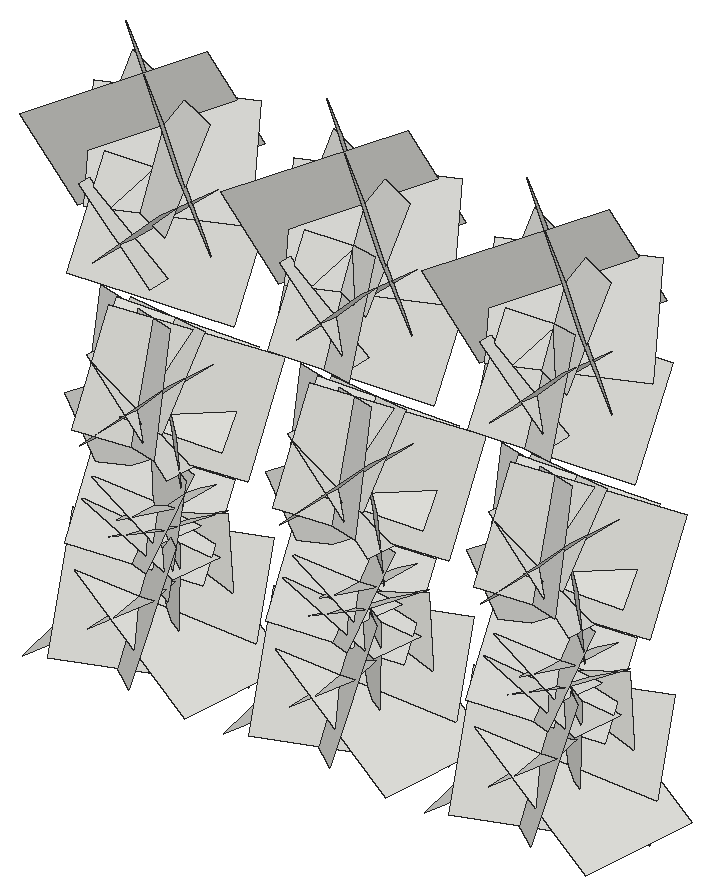
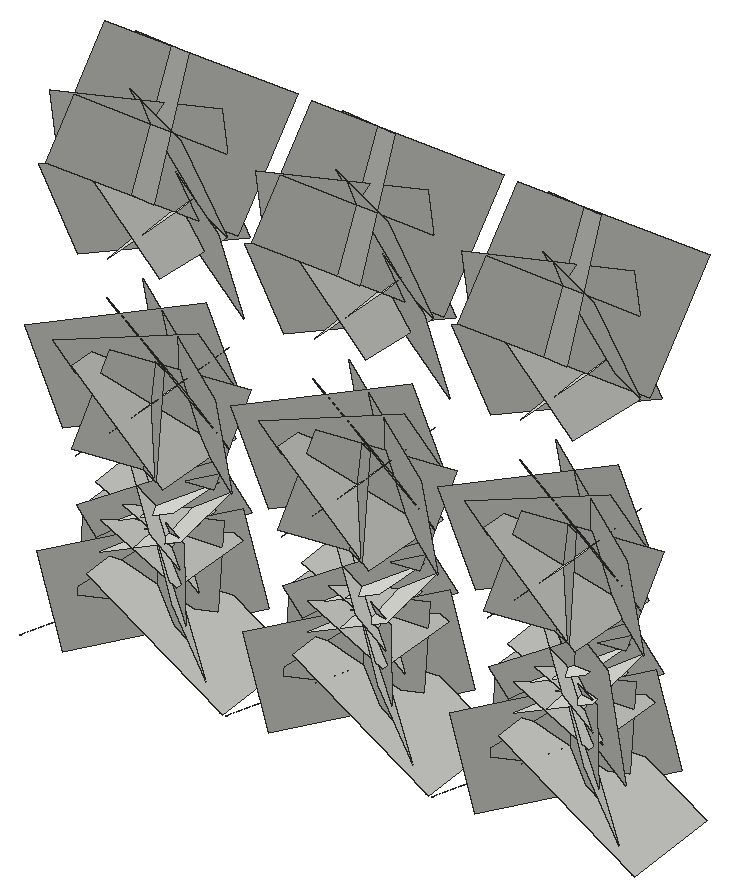
# SketchUp Ruby script. Lengths in inches.
U = 1.inch
M = Sketchup.active_model
def pt(a) = Geom::Point3d.new(a.map { |v| v * U })
def face(e, loops, mat)
  f = e.add_face(loops[0].map { |a| pt(a) })
  loops[1..].each { |l| e.add_face(l.map { |a| pt(a) }).erase! }
  f.material = f.back_material = mat if mat
  f
end
# faces: each face lists its corners as indices into pts; further lists are holes
def faces(e, pts, list, mat = nil) = list.each { |f| face(e, (f[0].is_a?(Array) ? f : [f]).map { |l| l.map { |i| pts[i] } }, mat) }
# xy, xz, yz: faces in a plane at the given z, y or x. An outline is a flat list of corners, or four numbers for a rectangle; further outlines are holes
def ring(l) = l.size == 4 ? [[l[0], l[1]], [l[2], l[1]], [l[2], l[3]], [l[0], l[3]]] : l.each_slice(2).to_a
def flat(e, list, mat, &to3) = list.each { |f| face(e, (f[0].is_a?(Array) ? f : [f]).map { |l| ring(l).map { |u, v| to3.(u, v) } }, mat) }
def xy(e, z, list, mat = nil) = flat(e, list, mat) { |x, y| [x, y, z] }
def xz(e, y, list, mat = nil) = flat(e, list, mat) { |x, z| [x, y, z] }
def yz(e, x, list, mat = nil) = flat(e, list, mat) { |y, z| [x, y, z] }
def lines(e, pts, list) = list.each { |a, b| e.add_line(pt(pts[a]), pt(pts[b])) }
# prism: a flat outline (further loops are holes) pulled along v
def prism(e, loops, v, mat = nil)
  f = face(e, loops, mat); d = Geom::Vector3d.new(v.map { |x| x * U })
  f.pushpull(f.normal.samedirection?(d) ? d.length : -d.length)
end
def box(e, o, s, mat = nil) = prism(e, [[o, [o[0] + s[0], o[1], o[2]], [o[0] + s[0], o[1] + s[1], o[2]], [o[0], o[1] + s[1], o[2]]]], [0, 0, s[2]], mat)
def at(x, y, z, deg = 0) = Geom::Transformation.translation(pt([x, y, z])) * Geom::Transformation.rotation(ORIGIN, Z_AXIS, deg.degrees)
def axes(o, x, y, z) = Geom::Transformation.new([*x, 0, *y, 0, *z, 0, *pt(o).to_a, 1])
def part(name) = M.definitions.add(name)
# library, detail: a bought-in or finely detailed component or shape, given as its bounding box
def library(name, o, s) = part(name).tap { |d| box(d.entities, o, s) }
def detail(e, o, s) = box(e.add_group.entities, o, s)
def put(e, d, t, mat = nil) = e.add_instance(d, t).tap { |i| i.material = mat if mat }
def group(e, t, mat = nil) = e.add_group.tap { |g| g.transformation = t; g.material = mat if mat }.entities
root = M.entities
c1 = part("Component\#6")
p = [[0.01,0,0],[0,3.24,4.54],[4.32,3.24,4.54],[4.33,0,0]]
faces(c1.entities,p,[[0,1,2,3]])
put(root,c1,axes([28.31,208.7,17.77],[-0.06939,0.44909,1.0594],[-0.12824,1.05255,-0.45366],[-1.21294,-0.13697,-0.01265]))
put(root,c1,axes([38.11,208.7,17.77],[-0.06939,0.44909,1.0594],[-0.12824,1.05255,-0.45366],[-1.21294,-0.13697,-0.01265]))
put(root,c1,axes([14.53,208.7,17.77],[0.06939,0.44909,1.0594],[0.12824,1.05255,-0.45366],[1.21294,-0.13697,-0.01265]))
put(root,c1,axes([24.34,208.7,17.77],[0.06939,0.44909,1.0594],[0.12824,1.05255,-0.45366],[1.21294,-0.13697,-0.01265]))
put(root,c1,axes([34.14,208.7,17.77],[0.06939,0.44909,1.0594],[0.12824,1.05255,-0.45366],[1.21294,-0.13697,-0.01265]))
put(root,c1,axes([18.5,207.55,1.43],[0.12288,0.50669,1.25804],[0.22547,1.24021,-0.51911],[-1.41983,0.2408,0.02645]))
put(root,c1,axes([14.53,207.55,1.43],[-0.12288,0.50669,1.25804],[-0.22547,1.24021,-0.51911],[1.41983,0.2408,0.02645]))
put(root,c1,axes([28.31,207.55,1.43],[0.12288,0.50669,1.25804],[0.22547,1.24021,-0.51911],[-1.41983,0.2408,0.02645]))
put(root,c1,axes([24.34,207.55,1.43],[-0.12288,0.50669,1.25804],[-0.22547,1.24021,-0.51911],[1.41983,0.2408,0.02645]))
put(root,c1,axes([38.11,207.55,1.43],[0.12288,0.50669,1.25804],[0.22547,1.24021,-0.51911],[-1.41983,0.2408,0.02645]))
put(root,c1,axes([34.14,207.55,1.43],[-0.12288,0.50669,1.25804],[-0.22547,1.24021,-0.51911],[1.41983,0.2408,0.02645]))
put(root,c1,axes([14.53,209.4375,21.31],[-0.06259,0.84258,-0.05617],[-0.1593,-0.0659,-0.83045],[0.88082,0.04795,-0.15418]))
put(root,c1,axes([18.5,209.4375,21.31],[0.06259,0.84258,-0.05617],[0.1593,-0.0659,-0.83045],[-0.88082,0.04795,-0.15418]))
put(root,c1,axes([24.34,209.4375,21.31],[-0.06259,0.84258,-0.05617],[-0.1593,-0.0659,-0.83045],[0.88082,0.04795,-0.15418]))
put(root,c1,axes([28.31,209.4375,21.31],[0.06259,0.84258,-0.05617],[0.1593,-0.0659,-0.83045],[-0.88082,0.04795,-0.15418]))
put(root,c1,axes([34.14,209.4375,21.31],[-0.06259,0.84258,-0.05617],[-0.1593,-0.0659,-0.83045],[0.88082,0.04795,-0.15418]))
put(root,c1,axes([38.11,209.4375,21.31],[0.06259,0.84258,-0.05617],[0.1593,-0.0659,-0.83045],[-0.88082,0.04795,-0.15418]))
put(root,c1,axes([18.5,209.66,7.46],[0.07333,0.81549,-0.13491],[-0.15326,-0.12136,-0.8077],[-0.86266,0.09088,0.13203]))
put(root,c1,axes([28.31,209.66,7.46],[0.07333,0.81549,-0.13491],[-0.15326,-0.12136,-0.8077],[-0.86266,0.09088,0.13203]))
put(root,c1,axes([38.11,209.66,7.46],[0.07333,0.81549,-0.13491],[-0.15326,-0.12136,-0.8077],[-0.86266,0.09088,0.13203]))
put(root,c1,axes([14.53,209.66,7.46],[-0.07333,0.81549,-0.13491],[0.15326,-0.12136,-0.8077],[0.86266,0.09088,0.13203]))
put(root,c1,axes([24.34,209.66,7.46],[-0.07333,0.81549,-0.13491],[0.15326,-0.12136,-0.8077],[0.86266,0.09088,0.13203]))
put(root,c1,axes([34.14,209.66,7.46],[-0.07333,0.81549,-0.13491],[0.15326,-0.12136,-0.8077],[0.86266,0.09088,0.13203]))
put(root,c1,axes([14.53,208.59,6.01],[-0.08926,0.55811,0.79685],[-0.15858,0.78289,-0.56414],[1.01897,0.17073,-0.01799]))
put(root,c1,axes([18.5,208.59,6.01],[0.08926,0.55811,0.79685],[0.15858,0.78289,-0.56414],[-1.01897,0.17073,-0.01799]))
put(root,c1,axes([24.34,208.59,6.01],[-0.08926,0.55811,0.79685],[-0.15858,0.78289,-0.56414],[1.01897,0.17073,-0.01799]))
put(root,c1,axes([28.31,208.59,6.01],[0.08926,0.55811,0.79685],[0.15858,0.78289,-0.56414],[-1.01897,0.17073,-0.01799]))
put(root,c1,axes([34.14,208.59,6.01],[-0.08926,0.55811,0.79685],[-0.15858,0.78289,-0.56414],[1.01897,0.17073,-0.01799]))
put(root,c1,axes([38.11,208.59,6.01],[0.08926,0.55811,0.79685],[0.15858,0.78289,-0.56414],[-1.01897,0.17073,-0.01799]))
put(root,c1,axes([18.5,209.05,10.75],[-0.11444,0.37825,1.13851],[-0.07236,1.13932,-0.38499],[-1.26962,-0.09903,-0.08068]))
put(root,c1,axes([14.53,209.05,10.75],[0.11444,0.37825,1.13851],[0.07236,1.13932,-0.38499],[1.26962,-0.09903,-0.08068]))
put(root,c1,axes([28.31,209.05,10.75],[-0.11444,0.37825,1.13851],[-0.07236,1.13932,-0.38499],[-1.26962,-0.09903,-0.08068]))
put(root,c1,axes([24.34,209.05,10.75],[0.11444,0.37825,1.13851],[0.07236,1.13932,-0.38499],[1.26962,-0.09903,-0.08068]))
put(root,c1,axes([38.11,209.05,10.75],[-0.11444,0.37825,1.13851],[-0.07236,1.13932,-0.38499],[-1.26962,-0.09903,-0.08068]))
put(root,c1,axes([34.14,209.05,10.75],[0.11444,0.37825,1.13851],[0.07236,1.13932,-0.38499],[1.26962,-0.09903,-0.08068]))
put(root,c1,axes([18.5,209.13,4.61],[-0.2016,1.24111,0.06484],[0.01549,0.06782,-1.25535],[-1.31728,-0.18915,-0.02468]))
put(root,c1,axes([14.53,209.13,4.61],[0.2016,1.24111,0.06484],[-0.01549,0.06782,-1.25535],[1.31728,-0.18915,-0.02468]))
put(root,c1,axes([28.31,209.13,4.61],[-0.2016,1.24111,0.06484],[0.01549,0.06782,-1.25535],[-1.31728,-0.18915,-0.02468]))
put(root,c1,axes([24.34,209.13,4.61],[0.2016,1.24111,0.06484],[-0.01549,0.06782,-1.25535],[1.31728,-0.18915,-0.02468]))
put(root,c1,axes([38.11,209.13,4.61],[-0.2016,1.24111,0.06484],[0.01549,0.06782,-1.25535],[-1.31728,-0.18915,-0.02468]))
put(root,c1,axes([34.14,209.13,4.61],[0.2016,1.24111,0.06484],[-0.01549,0.06782,-1.25535],[1.31728,-0.18915,-0.02468]))
put(root,c1,axes([14.53,210.26,8.16],[0.03239,0.64464,-0.05696],[0.08466,-0.06034,-0.64009],[0.68073,-0.02317,0.08231]))
put(root,c1,axes([18.5,210.26,8.16],[-0.03239,0.64464,-0.05696],[-0.08466,-0.06034,-0.64009],[-0.68073,-0.02317,0.08231]))
put(root,c1,axes([24.34,210.26,8.16],[0.03239,0.64464,-0.05696],[0.08466,-0.06034,-0.64009],[0.68073,-0.02317,0.08231]))
put(root,c1,axes([28.31,210.26,8.16],[-0.03239,0.64464,-0.05696],[-0.08466,-0.06034,-0.64009],[-0.68073,-0.02317,0.08231]))
put(root,c1,axes([34.14,210.26,8.16],[0.03239,0.64464,-0.05696],[0.08466,-0.06034,-0.64009],[0.68073,-0.02317,0.08231]))
put(root,c1,axes([38.11,210.26,8.16],[-0.03239,0.64464,-0.05696],[-0.08466,-0.06034,-0.64009],[-0.68073,-0.02317,0.08231]))
put(root,c1,axes([18.5,212.31,27.23],[0.13595,0.64817,-1.16375],[0.16935,-1.16817,-0.63303],[-1.40181,-0.07826,-0.18933]))
put(root,c1,axes([14.53,212.31,27.23],[-0.13595,0.64817,-1.16375],[-0.16935,-1.16817,-0.63303],[1.40181,-0.07826,-0.18933]))
put(root,c1,axes([28.31,212.31,27.23],[0.13595,0.64817,-1.16375],[0.16935,-1.16817,-0.63303],[-1.40181,-0.07826,-0.18933]))
put(root,c1,axes([24.34,212.31,27.23],[-0.13595,0.64817,-1.16375],[-0.16935,-1.16817,-0.63303],[1.40181,-0.07826,-0.18933]))
put(root,c1,axes([38.11,212.31,27.23],[0.13595,0.64817,-1.16375],[0.16935,-1.16817,-0.63303],[-1.40181,-0.07826,-0.18933]))
put(root,c1,axes([34.14,212.31,27.23],[-0.13595,0.64817,-1.16375],[-0.16935,-1.16817,-0.63303],[1.40181,-0.07826,-0.18933]))
put(root,c1,axes([18.5,209.54,11.71],[0.0382,0.56931,0.80625],[-0.18345,0.79793,-0.5557],[-1.03,-0.121,0.12888]))
put(root,c1,axes([14.53,209.54,11.71],[-0.0382,0.56931,0.80625],[0.18345,0.79793,-0.5557],[1.03,-0.121,0.12888]))
put(root,c1,axes([28.31,209.54,11.71],[0.0382,0.56931,0.80625],[-0.18345,0.79793,-0.5557],[-1.03,-0.121,0.12888]))
put(root,c1,axes([24.34,209.54,11.71],[-0.0382,0.56931,0.80625],[0.18345,0.79793,-0.5557],[1.03,-0.121,0.12888]))
put(root,c1,axes([38.11,209.54,11.71],[0.0382,0.56931,0.80625],[-0.18345,0.79793,-0.5557],[-1.03,-0.121,0.12888]))
put(root,c1,axes([34.14,209.54,11.71],[-0.0382,0.56931,0.80625],[0.18345,0.79793,-0.5557],[1.03,-0.121,0.12888]))
put(root,c1,axes([18.5,210.59,2.66],[0.04023,-0.02679,0.90097],[-0.06825,0.89939,0.02945],[-0.95301,-0.06554,0.03592]))
put(root,c1,axes([14.53,210.59,2.66],[-0.04023,-0.02679,0.90097],[0.06825,0.89939,0.02945],[0.95301,-0.06554,0.03592]))
put(root,c1,axes([28.31,210.59,2.66],[0.04023,-0.02679,0.90097],[-0.06825,0.89939,0.02945],[-0.95301,-0.06554,0.03592]))
put(root,c1,axes([24.34,210.59,2.66],[-0.04023,-0.02679,0.90097],[0.06825,0.89939,0.02945],[0.95301,-0.06554,0.03592]))
put(root,c1,axes([38.11,210.59,2.66],[0.04023,-0.02679,0.90097],[-0.06825,0.89939,0.02945],[-0.95301,-0.06554,0.03592]))
put(root,c1,axes([34.14,210.59,2.66],[-0.04023,-0.02679,0.90097],[0.06825,0.89939,0.02945],[0.95301,-0.06554,0.03592]))
put(root,c1,axes([14.53,210.86,7.98],[-0.16776,-0.30988,0.90566],[-0.16933,0.91363,0.28469],[1.00041,0.10267,0.20006]))
put(root,c1,axes([18.5,210.86,7.98],[0.16776,-0.30988,0.90566],[0.16933,0.91363,0.28469],[-1.00041,0.10267,0.20006]))
put(root,c1,axes([24.34,210.86,7.98],[-0.16776,-0.30988,0.90566],[-0.16933,0.91363,0.28469],[1.00041,0.10267,0.20006]))
put(root,c1,axes([28.31,210.86,7.98],[0.16776,-0.30988,0.90566],[0.16933,0.91363,0.28469],[-1.00041,0.10267,0.20006]))
put(root,c1,axes([34.14,210.86,7.98],[-0.16776,-0.30988,0.90566],[-0.16933,0.91363,0.28469],[1.00041,0.10267,0.20006]))
put(root,c1,axes([38.11,210.86,7.98],[0.16776,-0.30988,0.90566],[0.16933,0.91363,0.28469],[-1.00041,0.10267,0.20006]))
put(root,c1,axes([18.5,209.9375,13.64],[0.01722,0.9911,-0.0782],[0.18047,-0.07983,-0.97637],[-1.03826,0.00256,-0.17101]))
put(root,c1,axes([14.53,209.9375,13.64],[-0.01722,0.9911,-0.0782],[-0.18047,-0.07983,-0.97637],[1.03826,0.00256,-0.17101]))
put(root,c1,axes([28.31,209.9375,13.64],[0.01722,0.9911,-0.0782],[0.18047,-0.07983,-0.97637],[-1.03826,0.00256,-0.17101]))
put(root,c1,axes([24.34,209.9375,13.64],[-0.01722,0.9911,-0.0782],[-0.18047,-0.07983,-0.97637],[1.03826,0.00256,-0.17101]))
put(root,c1,axes([38.11,209.9375,13.64],[0.01722,0.9911,-0.0782],[0.18047,-0.07983,-0.97637],[-1.03826,0.00256,-0.17101]))
put(root,c1,axes([34.14,209.9375,13.64],[-0.01722,0.9911,-0.0782],[-0.18047,-0.07983,-0.97637],[1.03826,0.00256,-0.17101]))
put(root,c1,axes([18.5,209.74,20.23],[0.19527,0.38459,1.04089],[-0.21918,1.04855,-0.35083],[-1.15564,-0.13388,0.24241]))
put(root,c1,axes([28.31,209.74,20.23],[0.19527,0.38459,1.04089],[-0.21918,1.04855,-0.35083],[-1.15564,-0.13388,0.24241]))
put(root,c1,axes([38.11,209.74,20.23],[0.19527,0.38459,1.04089],[-0.21918,1.04855,-0.35083],[-1.15564,-0.13388,0.24241]))
put(root,c1,axes([14.53,209.74,20.23],[-0.19527,0.38459,1.04089],[0.21918,1.04855,-0.35083],[1.15564,-0.13388,0.24241]))
put(root,c1,axes([24.34,209.74,20.23],[-0.19527,0.38459,1.04089],[0.21918,1.04855,-0.35083],[1.15564,-0.13388,0.24241]))
put(root,c1,axes([34.14,209.74,20.23],[-0.19527,0.38459,1.04089],[0.21918,1.04855,-0.35083],[1.15564,-0.13388,0.24241]))
put(root,c1,axes([18.5,209.94,4.23],[0.07499,0.16237,1.17608],[-0.09639,1.17545,-0.15681],[-1.25477,-0.08059,0.08234]))
